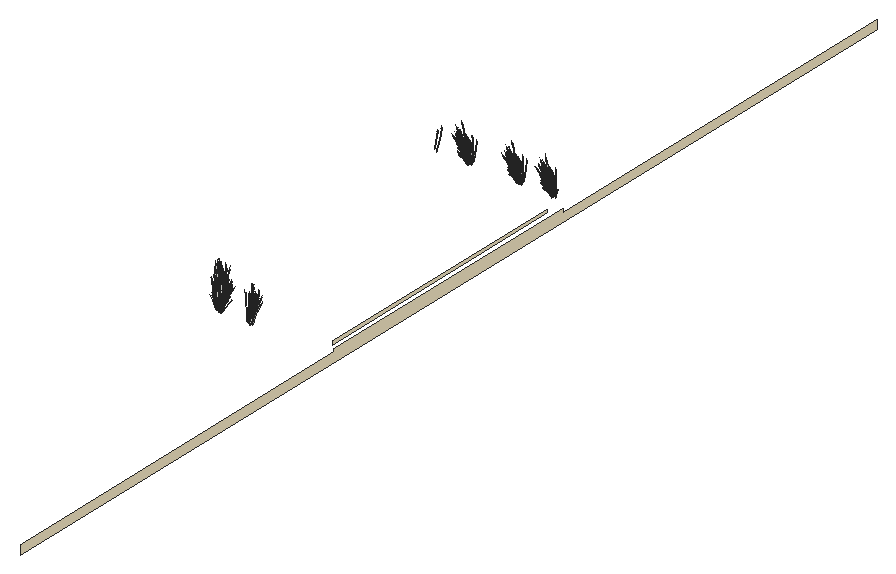
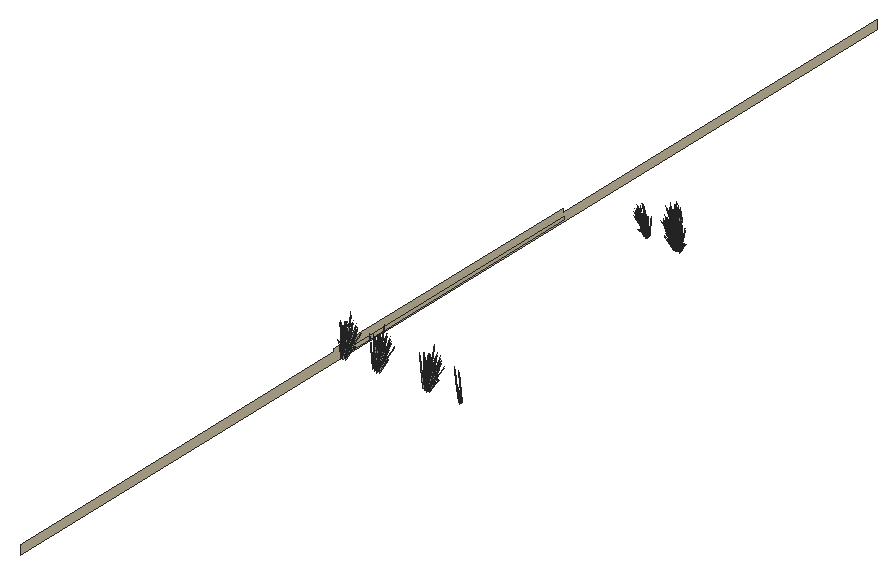
# SketchUp Ruby script. Lengths in inches.
U = 1.inch
M = Sketchup.active_model
def pt(a) = Geom::Point3d.new(a.map { |v| v * U })
def face(e, loops, mat)
  f = e.add_face(loops[0].map { |a| pt(a) })
  loops[1..].each { |l| e.add_face(l.map { |a| pt(a) }).erase! }
  f.material = f.back_material = mat if mat
  f
end
# faces: each face lists its corners as indices into pts; further lists are holes
def faces(e, pts, list, mat = nil) = list.each { |f| face(e, (f[0].is_a?(Array) ? f : [f]).map { |l| l.map { |i| pts[i] } }, mat) }
# xy, xz, yz: faces in a plane at the given z, y or x. An outline is a flat list of corners, or four numbers for a rectangle; further outlines are holes
def ring(l) = l.size == 4 ? [[l[0], l[1]], [l[2], l[1]], [l[2], l[3]], [l[0], l[3]]] : l.each_slice(2).to_a
def flat(e, list, mat, &to3) = list.each { |f| face(e, (f[0].is_a?(Array) ? f : [f]).map { |l| ring(l).map { |u, v| to3.(u, v) } }, mat) }
def xy(e, z, list, mat = nil) = flat(e, list, mat) { |x, y| [x, y, z] }
def xz(e, y, list, mat = nil) = flat(e, list, mat) { |x, z| [x, y, z] }
def yz(e, x, list, mat = nil) = flat(e, list, mat) { |y, z| [x, y, z] }
def lines(e, pts, list) = list.each { |a, b| e.add_line(pt(pts[a]), pt(pts[b])) }
# prism: a flat outline (further loops are holes) pulled along v
def prism(e, loops, v, mat = nil)
  f = face(e, loops, mat); d = Geom::Vector3d.new(v.map { |x| x * U })
  f.pushpull(f.normal.samedirection?(d) ? d.length : -d.length)
end
def box(e, o, s, mat = nil) = prism(e, [[o, [o[0] + s[0], o[1], o[2]], [o[0] + s[0], o[1] + s[1], o[2]], [o[0], o[1] + s[1], o[2]]]], [0, 0, s[2]], mat)
def at(x, y, z, deg = 0) = Geom::Transformation.translation(pt([x, y, z])) * Geom::Transformation.rotation(ORIGIN, Z_AXIS, deg.degrees)
def axes(o, x, y, z) = Geom::Transformation.new([*x, 0, *y, 0, *z, 0, *pt(o).to_a, 1])
def part(name) = M.definitions.add(name)
# library, detail: a bought-in or finely detailed component or shape, given as its bounding box
def library(name, o, s) = part(name).tap { |d| box(d.entities, o, s) }
def detail(e, o, s) = box(e.add_group.entities, o, s)
def put(e, d, t, mat = nil) = e.add_instance(d, t).tap { |i| i.material = mat if mat }
def group(e, t, mat = nil) = e.add_group.tap { |g| g.transformation = t; g.material = mat if mat }.entities
root = M.entities
M.materials.add("D01_Frost_White").color = [255, 242, 206]
M.materials.add("LightPink_Translucent").color = [144, 107, 117]
M.materials["LightPink_Translucent"].alpha = 0.75
c1 = part("blade")
p = [[2.15,0.21,22],[0,0.17,0],[0.09,0.45,0],[2.18,0.31,22],[2.29,0.31,22],[0.38,0.45,0],
  [2.48,0.24,33],[2.49,0.24,33],[2.48,0.22,33]]
faces(c1.entities,p,[[0,1,2,3],[4,5,2,3],[6,3,4,7],[8,0,3,6]])
c2 = part("seeds")
p = [[0.3,-0.1,1.38],[-0.01,-0.03,1.59],[-0.01,-0.03,0.03],[0.14,-0.07,-0.07],[0.29,-0.03,3],[0.15,0.01,3.11]]
faces(c2.entities,p,[[0,1,2,3],[1,0,4,5]],"LightPink_Translucent")
c3 = part("blade with seeds")
put(c3.entities,c1,at(0,0,0))
put(c3.entities,c2,axes([2.4,0.25,30.99],[1.5799,-0.05474,1.17369],[-0.12525,1.92788,0.29478],[-0.07173,-0.02425,1.56792]))
yz(root,846,[[288,0,468,2]],"D01_Frost_White")
yz(root,852,[[18,-6,738,-6,738,0,474,0,474,2,282,2,282,0,18,0]],"D01_Frost_White")
put(root,c3,axes([780.52,276.72,1.1],[-0.57436,-0.00261,-0.02488],[0,-0.36542,0.24971],[-0.01805,0.08319,0.79176]))
put(root,c3,axes([779.27,276.4,1.33],[0.51755,0.15601,-0.14548],[-0.2492,0.32927,-0.25001],[0.01626,0.08084,0.79854]))
put(root,c3,axes([801.53,276.82,1.33],[-0.2947,-0.01025,0.5253],[0.19462,-0.21779,0.29003],[0.11642,0.07737,0.41205]))
put(root,c3,axes([775.66,277.61,1.38],[0.19152,-0.14818,0.5743],[0.07557,0.23459,0.42196],[-0.13841,0.042,0.12649]))
put(root,c3,axes([780.27,277.34,2.26],[0.26148,0.20471,-0.17707],[-0.29857,0.19378,0.2286],[0.1517,0.02948,0.4374]))
put(root,c3,axes([780.4,276.77,1.01],[-0.32079,0.20399,-0.15489],[-0.32079,-0.20399,0.15489],[0,0.06571,0.69487]))
put(root,c3,axes([779.02,276.79,1.33],[0.05355,0.37308,-0.14548],[-0.55775,0.02256,-0.25001],[-0.09822,0.04969,0.79854]))
put(root,c3,axes([800.68,276.76,2.37],[-0.20887,0.2077,0.03215],[-0.29744,-0.12092,0.2531],[0.09616,0.06659,0.38595]))
put(root,c3,axes([780.14,277.42,2.37],[-0.02314,0.24862,0.03215],[-0.34943,-0.00682,0.2531],[0.13385,0.02602,0.38595]))
put(root,c3,axes([779.22,276.65,1.11],[-0.22297,0.29461,-0.2237],[-0.4633,-0.14179,0.10766],[0,0.06791,0.71822]))
put(root,c3,axes([776.38,276.97,2.26],[-0.40003,0.04673,-0.17707],[-0.10563,-0.26712,0.2286],[-0.11464,0.07175,0.4374]))
put(root,c3,axes([800.1875,277.46,2.82],[0.31757,-0.18757,-0.03244],[0.29098,0.20543,-0.14708],[0.02049,0.05821,0.48512]))
put(root,c3,axes([800.77,276.7,2.37],[-0.45708,0.07503,0.24001],[-0.07933,-0.29434,0.1979],[0.1075,0.08675,0.49665]))
put(root,c3,axes([780.17,277.34,2.37],[-0.33886,0.21544,0.24001],[-0.29224,-0.22879,0.1979],[0.15898,0.03974,0.49665]))
put(root,c3,axes([798.51,275.89,1.9375],[0.08557,-0.11238,0.85688],[0.35897,0.23257,0.06928],[-0.16194,0.14495,0.36631]))
put(root,c3,axes([800.57,276.29,1.3],[0.00811,-0.10838,0.71501],[0.38755,-0.12106,-0.15377],[0.11964,0.12972,0.3057]))
put(root,c3,axes([775.8,277.57,2.82],[0.40553,0.08728,-0.03244],[-0.12475,0.26862,-0.14708],[-0.06633,0.04078,0.48512]))
put(root,c3,axes([778.68,277.08,1.03],[-0.30954,0.24575,-0.31177],[-0.38452,-0.22284,-0.08182],[-0.12404,0.0613,0.68817]))
put(root,c3,axes([799.52,276.79,2.37],[-0.33863,0.11112,0.03215],[-0.16575,-0.20263,0.2531],[0.0327,0.08932,0.38595]))
put(root,c3,axes([798.61,276.52,2.26],[-0.31095,0.17214,-0.17707],[-0.29435,-0.19656,0.2286],[-0.04479,0.09987,0.4374]))
put(root,c3,axes([797.54,276.47,2.36],[-0.01142,0.0647,0.87472],[0.32418,0.22509,-0.13834],[-0.08487,0.10644,0.07015]))
put(root,c3,axes([798.57,276.33,2.7],[0.50507,0.0162,-0.06749],[-0.01381,0.30672,-0.3746],[-0.03508,0.11813,0.56919]))
put(root,c3,axes([779.09,277.59,2.53],[-0.07098,-0.26335,0.17707],[0.40574,-0.06954,-0.2286],[0.10898,0.07547,0.4374]))
put(root,c3,axes([799.51,276.67,2.52],[0.44971,-0.15222,-0.0608],[0.221,0.27017,-0.33747],[0.05933,0.11385,0.51278]))
put(root,c3,axes([779.23,277.49,1.17],[0.57533,0.10627,0.15378],[-0.14394,0.37986,-0.18246],[-0.09522,0.04754,0.82443]))
put(root,c3,axes([799.64,276.77,2.53],[-0.45283,-0.08548,0.26641],[0.15485,-0.28101,0.21967],[0.02721,0.11051,0.55128]))
put(root,c3,axes([779.19,277.75,1.01],[-0.4301,0.16348,-0.24825],[-0.25708,-0.29314,0],[-0.09796,0.03723,0.78752]))
put(root,c3,axes([780.62,276.78,1.01],[0,0.32696,-0.24825],[-0.51416,0,0],[0,0.07447,0.78752]))
put(root,c3,axes([779.33,276.82,1.9375],[-0.1707,-0.05633,0.85688],[0.35326,-0.23632,0.06928],[0.22018,0.10661,0.36631]))
put(root,c3,axes([798.81,277.19,1.38],[-0.01189,-0.19441,0.5743],[0.29719,0.13866,0.42196],[-0.05845,0.09266,0.12649]))
put(root,c3,axes([779.37,276.07,2.24],[-0.39711,-0.16988,0.69141],[0.41931,-0.2645,0.29833],[0.12812,0.1594,0.66832]))
put(root,c3,axes([799.59,276.73,0.75],[0.07437,-0.01779,0.88171],[0.44738,0.09793,-0.1347],[0.01308,0.11037,0.15018]))
put(root,c3,axes([776.5,276.79,2.52],[0.4251,0.18028,-0.0608],[-0.24491,0.26108,-0.33747],[-0.1201,0.09075,0.51278]))
put(root,c3,axes([779.97,277.46,1.38],[-0.25875,-0.09401,0.5743],[0.33411,-0.09552,0.42196],[0.09012,0.08091,0.12649]))
put(root,c3,axes([779.06,277.73,2.52],[0.27385,-0.27986,-0.0608],[0.39658,0.16123,-0.33747],[0.13785,0.07907,0.51278]))
put(root,c3,axes([798.92,276.44,2.5],[0.32898,0.21969,-0.2836],[-0.34753,0.1924,-0.21967],[-0.05006,0.11162,0.54264]))
put(root,c3,axes([777.08,276.71,1.9375],[0.11478,-0.10046,0.85688],[0.28982,0.27117,0.06928],[-0.19878,0.12349,0.36631]))
put(root,c3,axes([798.5625,276.77,1.41],[0.41748,-0.0579,0.03254],[0.09598,0.23326,-0.43152],[-0.02647,0.11808,0.3868]))
put(root,c3,axes([799.9,276.66,2.34],[0.45175,0.08196,-0.25549],[-0.15485,0.28101,-0.1979],[0.04142,0.11314,0.48886]))
put(root,c3,axes([800.15,276.07,1.9375],[-0.10505,-0.10498,0.85688],[0.48542,-0.08838,0.06928],[0.10971,0.1648,0.36631]))
put(root,c3,axes([776.71,277,2.34],[0.11806,0.29854,-0.25549],[-0.44709,0.05222,-0.1979],[-0.12812,0.08019,0.48886]))
put(root,c3,axes([777.25,277.35,2.53],[0.31095,-0.17214,0.17707],[0.29435,0.19656,-0.2286],[-0.04479,0.09987,0.4374]))
put(root,c3,axes([779.58,277.7,1.1875],[0.28732,0.32763,0],[-0.4807,0.18271,-0.25804],[-0.10948,0.04161,0.81856]))
put(root,c3,axes([778.7,277.96,2.35],[0.00136,-0.03958,0.88692],[0.39383,-0.17464,-0.08381],[0.1368,0.06234,0.15695]))
put(root,c3,axes([799.6875,276.83,2.26],[-0.13855,0.25143,-0.17707],[-0.4042,-0.07334,0.2286],[0.03706,0.10123,0.4374]))
put(root,c3,axes([780.04,277.81,0.75],[0.03348,-0.0472,0.88171],[0.42153,-0.13902,-0.1347],[0.12779,0.07195,0.15018]))
put(root,c3,axes([779.34,276.4,1.42],[-0.01255,-0.30784,0.70636],[0.56816,0.0798,0.29908],[-0.13438,0.16845,0.66675]))
put(root,c3,axes([779.48,276.73,1.05],[0.16851,0.29936,-0.34606],[-0.4854,0.10781,-0.09083],[0.01863,0.10137,0.76386]))
put(root,c3,axes([776.97,277.5,2.37],[-0.37765,-0.01523,0.03215],[0.01035,-0.23004,0.2531],[-0.03952,0.08812,0.38595]))
put(root,c3,axes([776.17,277.77,0.75],[0.06164,0.03267,0.88171],[0.10452,0.30266,-0.1347],[-0.13662,0.06454,0.15018]))
put(root,c3,axes([777.09,277.52,2.37],[-0.32725,-0.22308,0.24001],[0.34753,-0.1924,0.1979],[-0.06036,0.10466,0.49665]))
put(root,c3,axes([779.38,277.59,2.34],[0.45348,-0.07772,-0.25549],[0.07933,0.29434,-0.1979],[0.1218,0.08435,0.48886]))
put(root,c3,axes([798.82,276.34,2.67],[-0.01196,0.30243,-0.3943],[-0.50354,-0.02031,0.04758],[-0.05314,0.12813,0.55778]))
put(root,c3,axes([797.5,277.14,2.35],[0.05214,-0.01974,0.88692],[0.43092,0.1313,-0.08381],[-0.01013,0.10932,0.15695]))
put(root,c3,axes([778.125,277.63,2.53],[0.13855,-0.25143,0.17707],[0.4042,0.07334,-0.2286],[0.03706,0.10123,0.4374]))
put(root,c3,axes([799.29,276.13,1.9375],[-0.01125,-0.12549,0.85688],[0.48751,0.08325,0.06928],[-0.03015,0.17883,0.36631]))
put(root,c3,axes([780.01,277.88,1.33],[-0.2947,-0.01025,0.5253],[0.19462,-0.21779,0.29003],[0.11642,0.07737,0.41205]))
put(root,c3,axes([779.16,277.83,2.37],[-0.20887,0.2077,0.03215],[-0.29744,-0.12092,0.2531],[0.09616,0.06659,0.38595]))
put(root,c3,axes([799.73,276.6,2.49],[0.21934,0.26585,-0.35523],[-0.45151,0.14816,0.04287],[0.05129,0.12845,0.5025]))
put(root,c3,axes([778.67,278.53,2.82],[0.31757,-0.18757,-0.03244],[0.29098,0.20543,-0.14708],[0.02049,0.05821,0.48512]))
put(root,c3,axes([779.25,277.77,2.37],[-0.45708,0.07503,0.24001],[-0.07933,-0.29434,0.1979],[0.1075,0.08675,0.49665]))
put(root,c3,axes([798.46,277.02,1.3],[0.14502,-0.05158,0.71501],[0.35805,0.15552,-0.15377],[-0.10657,0.13457,0.3057]))
put(root,c3,axes([799.4,277.27,2.36],[0.05825,0.05265,0.87472],[0.47011,0.02068,-0.13834],[0.04727,0.11612,0.07015]))
put(root,c3,axes([776.99,276.96,1.9375],[0.08557,-0.11238,0.85688],[0.35897,0.23257,0.06928],[-0.16194,0.14495,0.36631]))
put(root,c3,axes([779.04,277.36,1.3],[0.00811,-0.10838,0.71501],[0.38755,-0.12106,-0.15377],[0.11964,0.12972,0.3057]))
put(root,c3,axes([778,277.86,2.37],[-0.33863,0.11112,0.03215],[-0.16575,-0.20263,0.2531],[0.0327,0.08932,0.38595]))
put(root,c3,axes([777.09,277.59,2.26],[-0.31095,0.17214,-0.17707],[-0.29435,-0.19656,0.2286],[-0.04479,0.09987,0.4374]))
put(root,c3,axes([776.02,277.54,2.36],[-0.01142,0.0647,0.87472],[0.32418,0.22509,-0.13834],[-0.08487,0.10644,0.07015]))
put(root,c3,axes([777.05,277.39,2.7],[0.50507,0.0162,-0.06749],[-0.01381,0.30672,-0.3746],[-0.03508,0.11813,0.56919]))
put(root,c3,axes([777.99,277.74,2.52],[0.44971,-0.15222,-0.0608],[0.221,0.27017,-0.33747],[0.05933,0.11385,0.51278]))
put(root,c3,axes([778.12,277.84,2.53],[-0.45283,-0.08548,0.26641],[0.15485,-0.28101,0.21967],[0.02721,0.11051,0.55128]))
put(root,c3,axes([777.29,278.26,1.38],[-0.01189,-0.19441,0.5743],[0.29719,0.13866,0.42196],[-0.05845,0.09266,0.12649]))
put(root,c3,axes([778.07,277.8,0.75],[0.07437,-0.01779,0.88171],[0.44738,0.09793,-0.1347],[0.01308,0.11037,0.15018]))
put(root,c3,axes([798.65,276.77,1.68],[0.0101,-0.16879,0.77173],[0.45413,0.08915,0.10664],[-0.03935,0.17989,0.36441]))
put(root,c3,axes([777.4,277.51,2.5],[0.32898,0.21969,-0.2836],[-0.34753,0.1924,-0.21967],[-0.05006,0.11162,0.54264]))
put(root,c3,axes([777.04,277.84,1.41],[0.41748,-0.0579,0.03254],[0.09598,0.23326,-0.43152],[-0.02647,0.11808,0.3868]))
put(root,c3,axes([778.375,277.72,2.34],[0.45175,0.08196,-0.25549],[-0.15485,0.28101,-0.1979],[0.04142,0.11314,0.48886]))
put(root,c3,axes([778.63,277.14,1.9375],[-0.10505,-0.10498,0.85688],[0.48542,-0.08838,0.06928],[0.10971,0.1648,0.36631]))
put(root,c3,axes([778.17,277.9,2.26],[-0.13855,0.25143,-0.17707],[-0.4042,-0.07334,0.2286],[0.03706,0.10123,0.4374]))
put(root,c3,axes([777.3,277.41,2.67],[-0.01196,0.30243,-0.3943],[-0.50354,-0.02031,0.04758],[-0.05314,0.12813,0.55778]))
put(root,c3,axes([775.98,278.2,2.35],[0.05214,-0.01974,0.88692],[0.43092,0.1313,-0.08381],[-0.01013,0.10932,0.15695]))
put(root,c3,axes([777.77,277.2,1.9375],[-0.01125,-0.12549,0.85688],[0.48751,0.08325,0.06928],[-0.03015,0.17883,0.36631]))
put(root,c3,axes([778.21,277.67,2.49],[0.21934,0.26585,-0.35523],[-0.45151,0.14816,0.04287],[0.05129,0.12845,0.5025]))
put(root,c3,axes([776.94,278.09,1.3],[0.14502,-0.05158,0.71501],[0.35805,0.15552,-0.15377],[-0.10657,0.13457,0.3057]))
put(root,c3,axes([777.88,278.34,2.36],[0.05825,0.05265,0.87472],[0.47011,0.02068,-0.13834],[0.04727,0.11612,0.07015]))
put(root,c3,axes([777.13,277.84,1.68],[0.0101,-0.16879,0.77173],[0.45413,0.08915,0.10664],[-0.03935,0.17989,0.36441]))
put(root,c3,axes([783.61,479.97,3.9375],[0.10505,0.10498,0.85688],[-0.48542,0.08838,0.06928],[-0.10971,-0.1648,0.36631]))
put(root,c3,axes([817.3,479.97,3.9375],[0.10505,0.10498,0.85688],[-0.48542,0.08838,0.06928],[-0.10971,-0.1648,0.36631]))
put(root,c3,axes([839.89,479.97,3.9375],[0.10505,0.10498,0.85688],[-0.48542,0.08838,0.06928],[-0.10971,-0.1648,0.36631]))
put(root,c3,axes([784.41,479.28,4.36],[-0.07029,-0.04584,0.87472],[-0.46908,0.02906,-0.13834],[-0.07486,-0.10965,0.07015]))
put(root,c3,axes([818.1,479.28,4.36],[-0.07029,-0.04584,0.87472],[-0.46908,0.02906,-0.13834],[-0.07486,-0.10965,0.07015]))
put(root,c3,axes([840.69,479.28,4.36],[-0.07029,-0.04584,0.87472],[-0.46908,0.02906,-0.13834],[-0.07486,-0.10965,0.07015]))
put(root,c3,axes([785.5,479.82,3.3],[-0.13063,0.06618,0.71501],[-0.39122,-0.11583,-0.15377],[0.07252,-0.14406,0.3057]))
put(root,c3,axes([819.19,479.82,3.3],[-0.13063,0.06618,0.71501],[-0.39122,-0.11583,-0.15377],[0.07252,-0.14406,0.3057]))
put(root,c3,axes([841.78,479.82,3.3],[-0.13063,0.06618,0.71501],[-0.39122,-0.11583,-0.15377],[0.07252,-0.14406,0.3057]))
put(root,c3,axes([784.9,480.05,4.49],[-0.21934,-0.26585,-0.35523],[0.45151,-0.14816,0.04287],[-0.05129,-0.12845,0.5025]))
put(root,c3,axes([818.6,480.05,4.49],[-0.21934,-0.26585,-0.35523],[0.45151,-0.14816,0.04287],[-0.05129,-0.12845,0.5025]))
put(root,c3,axes([841.18,480.05,4.49],[-0.21934,-0.26585,-0.35523],[0.45151,-0.14816,0.04287],[-0.05129,-0.12845,0.5025]))
put(root,c3,axes([783.47,479.69,3.3],[-0.02783,0.10696,0.71501],[-0.40683,0.08954,-0.15377],[-0.0951,-0.13825,0.3057]))
put(root,c3,axes([817.17,479.69,3.3],[-0.02783,0.10696,0.71501],[-0.40683,0.08954,-0.15377],[-0.0951,-0.13825,0.3057]))
put(root,c3,axes([839.76,479.69,3.3],[-0.02783,0.10696,0.71501],[-0.40683,0.08954,-0.15377],[-0.0951,-0.13825,0.3057]))
put(root,c3,axes([784.52,479.46,2.75],[-0.07708,0.01178,0.88171],[-0.42627,-0.1326,-0.1347],[0.00715,-0.1106,0.15018]))
put(root,c3,axes([818.22,479.46,2.75],[-0.07708,0.01178,0.88171],[-0.42627,-0.1326,-0.1347],[0.00715,-0.1106,0.15018]))
put(root,c3,axes([840.8,479.46,2.75],[-0.07708,0.01178,0.88171],[-0.42627,-0.1326,-0.1347],[0.00715,-0.1106,0.15018]))
put(root,c3,axes([785.8125,480.31,4.49],[0.01196,-0.30243,-0.35523],[0.50354,0.02031,0.04287],[0.05314,-0.12813,0.5025]))
put(root,c3,axes([819.51,480.31,4.49],[0.01196,-0.30243,-0.35523],[0.50354,0.02031,0.04287],[0.05314,-0.12813,0.5025]))
put(root,c3,axes([842.1,480.31,4.49],[0.01196,-0.30243,-0.35523],[0.50354,0.02031,0.04287],[0.05314,-0.12813,0.5025]))
put(root,c3,axes([786.52,479.84,4.36],[-0.00444,-0.06507,0.87472],[-0.37468,-0.18807,-0.13834],[0.05793,-0.114,0.07015]))
put(root,c3,axes([820.21,479.84,4.36],[-0.00444,-0.06507,0.87472],[-0.37468,-0.18807,-0.13834],[0.05793,-0.114,0.07015]))
put(root,c3,axes([842.8,479.84,4.36],[-0.00444,-0.06507,0.87472],[-0.37468,-0.18807,-0.13834],[0.05793,-0.114,0.07015]))
put(root,c3,axes([784.94,479.82,4.26],[0.13855,-0.25143,-0.17707],[0.4042,0.07334,0.2286],[-0.03706,-0.10123,0.4374]))
put(root,c3,axes([818.64,479.82,4.26],[0.13855,-0.25143,-0.17707],[0.4042,0.07334,0.2286],[-0.03706,-0.10123,0.4374]))
put(root,c3,axes([841.22,479.82,4.26],[0.13855,-0.25143,-0.17707],[0.4042,0.07334,0.2286],[-0.03706,-0.10123,0.4374]))
put(root,c3,axes([761.49,480.16,3.9375],[-0.08557,0.11238,0.85688],[-0.35897,-0.23257,0.06928],[0.16194,-0.14495,0.36631]))
put(root,c3,axes([785.25,480.16,3.9375],[-0.08557,0.11238,0.85688],[-0.35897,-0.23257,0.06928],[0.16194,-0.14495,0.36631]))
put(root,c3,axes([818.94,480.16,3.9375],[-0.08557,0.11238,0.85688],[-0.35897,-0.23257,0.06928],[0.16194,-0.14495,0.36631]))
put(root,c3,axes([841.53,480.16,3.9375],[-0.08557,0.11238,0.85688],[-0.35897,-0.23257,0.06928],[0.16194,-0.14495,0.36631]))
put(root,c3,axes([786.42,479.6,4.35],[-0.04667,0.02497,0.88692],[-0.45726,-0.08426,-0.08381],[-0.01655,-0.10898,0.15695]))
put(root,c3,axes([820.11,479.6,4.35],[-0.04667,0.02497,0.88692],[-0.45726,-0.08426,-0.08381],[-0.01655,-0.10898,0.15695]))
put(root,c3,axes([842.7,479.6,4.35],[-0.04667,0.02497,0.88692],[-0.45726,-0.08426,-0.08381],[-0.01655,-0.10898,0.15695]))
put(root,c3,axes([784.74,480,4.34],[-0.45175,-0.08196,-0.25549],[0.15485,-0.28101,-0.1979],[-0.04142,-0.11314,0.48886]))
put(root,c3,axes([818.43,480,4.34],[-0.45175,-0.08196,-0.25549],[0.15485,-0.28101,-0.1979],[-0.04142,-0.11314,0.48886]))
put(root,c3,axes([841.02,480,4.34],[-0.45175,-0.08196,-0.25549],[0.15485,-0.28101,-0.1979],[-0.04142,-0.11314,0.48886]))
put(root,c3,axes([785.02,479.29,3.38],[0.05895,0.19066,0.5743],[-0.32704,-0.1056,0.42196],[0.03519,-0.09762,0.12649]))
put(root,c3,axes([818.71,479.29,3.38],[0.05895,0.19066,0.5743],[-0.32704,-0.1056,0.42196],[0.03519,-0.09762,0.12649]))
put(root,c3,axes([841.3,479.29,3.38],[0.05895,0.19066,0.5743],[-0.32704,-0.1056,0.42196],[0.03519,-0.09762,0.12649]))
put(root,c3,axes([785.71,480.21,4.34],[-0.32898,-0.21969,-0.25549],[0.34753,-0.1924,-0.1979],[0.05006,-0.11162,0.48886]))
put(root,c3,axes([819.41,480.21,4.34],[-0.32898,-0.21969,-0.25549],[0.34753,-0.1924,-0.1979],[0.05006,-0.11162,0.48886]))
put(root,c3,axes([841.99,480.21,4.34],[-0.32898,-0.21969,-0.25549],[0.34753,-0.1924,-0.1979],[0.05006,-0.11162,0.48886]))
put(root,c3,axes([783.93,479.125,4.35],[-0.00857,0.03919,0.88692],[-0.42284,0.14223,-0.08381],[-0.12443,-0.0727,0.15695]))
put(root,c3,axes([817.62,479.125,4.35],[-0.00857,0.03919,0.88692],[-0.42284,0.14223,-0.08381],[-0.12443,-0.0727,0.15695]))
put(root,c3,axes([840.21,479.125,4.35],[-0.00857,0.03919,0.88692],[-0.42284,0.14223,-0.08381],[-0.12443,-0.0727,0.15695]))
put(root,c3,axes([783.83,479.82,4.55],[0.51193,-0.08404,0.26881],[0.08885,0.32966,0.22165],[-0.1204,-0.09716,0.55625]))
put(root,c3,axes([817.53,479.82,4.55],[0.51193,-0.08404,0.26881],[0.08885,0.32966,0.22165],[-0.1204,-0.09716,0.55625]))
put(root,c3,axes([840.12,479.82,4.55],[0.51193,-0.08404,0.26881],[0.08885,0.32966,0.22165],[-0.1204,-0.09716,0.55625]))
put(root,c3,axes([784.99,479.88,4.37],[0.45283,0.08548,0.24001],[-0.15485,0.28101,0.1979],[-0.02721,-0.11051,0.49665]))
put(root,c3,axes([818.6875,479.88,4.37],[0.45283,0.08548,0.24001],[-0.15485,0.28101,0.1979],[-0.02721,-0.11051,0.49665]))
put(root,c3,axes([841.27,479.88,4.37],[0.45283,0.08548,0.24001],[-0.15485,0.28101,0.1979],[-0.02721,-0.11051,0.49665]))
put(root,c3,axes([785.12,479.98,4.52],[-0.44971,0.15222,-0.0608],[-0.221,-0.27017,-0.33747],[-0.05933,-0.11385,0.51278]))
put(root,c3,axes([818.82,479.98,4.52],[-0.44971,0.15222,-0.0608],[-0.221,-0.27017,-0.33747],[-0.05933,-0.11385,0.51278]))
put(root,c3,axes([841.4,479.98,4.52],[-0.44971,0.15222,-0.0608],[-0.221,-0.27017,-0.33747],[-0.05933,-0.11385,0.51278]))
put(root,c3,axes([786.06,480.32,4.52],[-0.50507,-0.0162,-0.0608],[0.01381,-0.30672,-0.33747],[0.03508,-0.11813,0.51278]))
put(root,c3,axes([819.75,480.32,4.52],[-0.50507,-0.0162,-0.0608],[0.01381,-0.30672,-0.33747],[0.03508,-0.11813,0.51278]))
put(root,c3,axes([842.34,480.32,4.52],[-0.50507,-0.0162,-0.0608],[0.01381,-0.30672,-0.33747],[0.03508,-0.11813,0.51278]))
put(root,c3,axes([786.02,480.13,4.26],[0.31095,-0.17214,-0.17707],[0.29435,0.19656,0.2286],[0.04479,-0.09987,0.4374]))
put(root,c3,axes([819.72,480.13,4.26],[0.31095,-0.17214,-0.17707],[0.29435,0.19656,0.2286],[0.04479,-0.09987,0.4374]))
put(root,c3,axes([842.3,480.13,4.26],[0.31095,-0.17214,-0.17707],[0.29435,0.19656,0.2286],[0.04479,-0.09987,0.4374]))
put(root,c3,axes([783.33,479.52,3.38],[0.23972,0.1138,0.5743],[-0.34912,0.06841,0.42196],[-0.0747,-0.08746,0.12649]))
put(root,c3,axes([817.03,479.52,3.38],[0.23972,0.1138,0.5743],[-0.34912,0.06841,0.42196],[-0.0747,-0.08746,0.12649]))
put(root,c3,axes([839.62,479.52,3.38],[0.23972,0.1138,0.5743],[-0.34912,0.06841,0.42196],[-0.0747,-0.08746,0.12649]))
put(root,c3,axes([785.11,479.86,4.37],[0.33863,-0.11112,0.03215],[0.16575,0.20263,0.2531],[-0.0327,-0.08932,0.38595]))
put(root,c3,axes([818.81,479.86,4.37],[0.33863,-0.11112,0.03215],[0.16575,0.20263,0.2531],[-0.0327,-0.08932,0.38595]))
put(root,c3,axes([841.39,479.86,4.37],[0.33863,-0.11112,0.03215],[0.16575,0.20263,0.2531],[-0.0327,-0.08932,0.38595]))
put(root,c3,axes([783.91,480.125,4.49],[-0.39186,-0.15803,-0.35523],[0.27849,-0.27693,0.04287],[-0.14198,-0.09436,0.5025]))
put(root,c3,axes([817.61,480.125,4.49],[-0.39186,-0.15803,-0.35523],[0.27849,-0.27693,0.04287],[-0.14198,-0.09436,0.5025]))
put(root,c3,axes([840.19,480.125,4.49],[-0.39186,-0.15803,-0.35523],[0.27849,-0.27693,0.04287],[-0.14198,-0.09436,0.5025]))
put(root,c3,axes([783.78,479.92,4.26],[-0.07098,-0.26335,-0.17707],[0.40574,-0.06954,0.2286],[-0.10898,-0.07547,0.4374]))
put(root,c3,axes([817.47,479.92,4.26],[-0.07098,-0.26335,-0.17707],[0.40574,-0.06954,0.2286],[-0.10898,-0.07547,0.4374]))
put(root,c3,axes([840.06,479.92,4.26],[-0.07098,-0.26335,-0.17707],[0.40574,-0.06954,0.2286],[-0.10898,-0.07547,0.4374]))
put(root,c3,axes([783.95,479.89,4.37],[0.20887,-0.2077,0.03215],[0.29744,0.12092,0.2531],[-0.09616,-0.06659,0.38595]))
put(root,c3,axes([817.65,479.89,4.37],[0.20887,-0.2077,0.03215],[0.29744,0.12092,0.2531],[-0.09616,-0.06659,0.38595]))
put(root,c3,axes([840.23,479.89,4.37],[0.20887,-0.2077,0.03215],[0.29744,0.12092,0.2531],[-0.09616,-0.06659,0.38595]))
put(root,c3,axes([783.14,479.86,2.75],[-0.04451,0.04307,0.88171],[-0.44986,0.09286,-0.1347],[-0.10868,-0.08448,0.15018]))
put(root,c3,axes([816.84,479.86,2.75],[-0.04451,0.04307,0.88171],[-0.44986,0.09286,-0.1347],[-0.10868,-0.08448,0.15018]))
put(root,c3,axes([839.43,479.86,2.75],[-0.04451,0.04307,0.88171],[-0.44986,0.09286,-0.1347],[-0.10868,-0.08448,0.15018]))
put(root,c3,axes([783.89,481.05,3.05],[-0.18873,-0.33528,-0.34918],[0.54365,-0.12075,-0.09164],[-0.02086,-0.11353,0.77075]))
put(root,c3,axes([817.58,481.05,3.05],[-0.18873,-0.33528,-0.34918],[0.54365,-0.12075,-0.09164],[-0.02086,-0.11353,0.77075]))
put(root,c3,axes([840.17,481.05,3.05],[-0.18873,-0.33528,-0.34918],[0.54365,-0.12075,-0.09164],[-0.02086,-0.11353,0.77075]))
put(root,c3,axes([782.9,480.3,3.9375],[0.1707,0.05633,0.85688],[-0.35326,0.23632,0.06928],[-0.22018,-0.10661,0.36631]))
put(root,c3,axes([816.6,480.3,3.9375],[0.1707,0.05633,0.85688],[-0.35326,0.23632,0.06928],[-0.22018,-0.10661,0.36631]))
put(root,c3,axes([839.19,480.3,3.9375],[0.1707,0.05633,0.85688],[-0.35326,0.23632,0.06928],[-0.22018,-0.10661,0.36631]))
put(root,c3,axes([762.65,480.02,2.75],[-0.06878,-0.02576,0.88171],[-0.17668,-0.28776,-0.1347],[0.11919,-0.07809,0.15018]))
put(root,c3,axes([786.41,480.02,2.75],[-0.06878,-0.02576,0.88171],[-0.17668,-0.28776,-0.1347],[0.11919,-0.07809,0.15018]))
put(root,c3,axes([820.1,480.02,2.75],[-0.06878,-0.02576,0.88171],[-0.17668,-0.28776,-0.1347],[0.11919,-0.07809,0.15018]))
put(root,c3,axes([842.69,480.02,2.75],[-0.06878,-0.02576,0.88171],[-0.17668,-0.28776,-0.1347],[0.11919,-0.07809,0.15018]))
put(root,c3,axes([784.99,480.09,4.53],[-0.13855,0.25143,0.17707],[-0.4042,-0.07334,-0.2286],[-0.03706,-0.10123,0.4374]))
put(root,c3,axes([818.68,480.09,4.53],[-0.13855,0.25143,0.17707],[-0.4042,-0.07334,-0.2286],[-0.03706,-0.10123,0.4374]))
put(root,c3,axes([841.27,480.09,4.53],[-0.13855,0.25143,0.17707],[-0.4042,-0.07334,-0.2286],[-0.03706,-0.10123,0.4374]))
put(root,c3,axes([783.73,480.13,4.34],[-0.45348,0.07772,-0.25549],[-0.07933,-0.29434,-0.1979],[-0.1218,-0.08435,0.48886]))
put(root,c3,axes([817.42,480.13,4.34],[-0.45348,0.07772,-0.25549],[-0.07933,-0.29434,-0.1979],[-0.1218,-0.08435,0.48886]))
put(root,c3,axes([840.01,480.13,4.34],[-0.45348,0.07772,-0.25549],[-0.07933,-0.29434,-0.1979],[-0.1218,-0.08435,0.48886]))
put(root,c3,axes([786.02,480.19,4.37],[0.32725,0.22308,0.24001],[-0.34753,0.1924,0.1979],[0.06036,-0.10466,0.49665]))
put(root,c3,axes([819.72,480.19,4.37],[0.32725,0.22308,0.24001],[-0.34753,0.1924,0.1979],[0.06036,-0.10466,0.49665]))
put(root,c3,axes([842.3,480.19,4.37],[0.32725,0.22308,0.24001],[-0.34753,0.1924,0.1979],[0.06036,-0.10466,0.49665]))
put(root,c3,axes([784.05,479.87,4.72],[-0.30671,0.31344,-0.0681],[-0.44417,-0.18058,-0.37797],[-0.1544,-0.08856,0.57432]))
put(root,c3,axes([817.74,479.87,4.72],[-0.30671,0.31344,-0.0681],[-0.44417,-0.18058,-0.37797],[-0.1544,-0.08856,0.57432]))
put(root,c3,axes([840.33,479.87,4.72],[-0.30671,0.31344,-0.0681],[-0.44417,-0.18058,-0.37797],[-0.1544,-0.08856,0.57432]))
put(root,c3,axes([786.14,480.22,4.37],[0.37765,0.01523,0.03215],[-0.01035,0.23004,0.2531],[0.03952,-0.08812,0.38595]))
put(root,c3,axes([819.84,480.22,4.37],[0.37765,0.01523,0.03215],[-0.01035,0.23004,0.2531],[0.03952,-0.08812,0.38595]))
put(root,c3,axes([842.42,480.22,4.37],[0.37765,0.01523,0.03215],[-0.01035,0.23004,0.2531],[0.03952,-0.08812,0.38595]))
put(root,c3,axes([785.86,480.37,4.53],[-0.31095,0.17214,0.17707],[-0.29435,-0.19656,-0.2286],[0.04479,-0.09987,0.4374]))
put(root,c3,axes([819.55,480.37,4.53],[-0.31095,0.17214,0.17707],[-0.29435,-0.19656,-0.2286],[0.04479,-0.09987,0.4374]))
put(root,c3,axes([842.14,480.37,4.53],[-0.31095,0.17214,0.17707],[-0.29435,-0.19656,-0.2286],[0.04479,-0.09987,0.4374]))
put(root,c3,axes([762.65,480.84,4.49],[0.24005,-0.25798,-0.35523],[0.42065,0.18334,0.04287],[0.14333,-0.09347,0.5025]))
put(root,c3,axes([786.41,480.84,4.49],[0.24005,-0.25798,-0.35523],[0.42065,0.18334,0.04287],[0.14333,-0.09347,0.5025]))
put(root,c3,axes([820.1,480.84,4.49],[0.24005,-0.25798,-0.35523],[0.42065,0.18334,0.04287],[0.14333,-0.09347,0.5025]))
